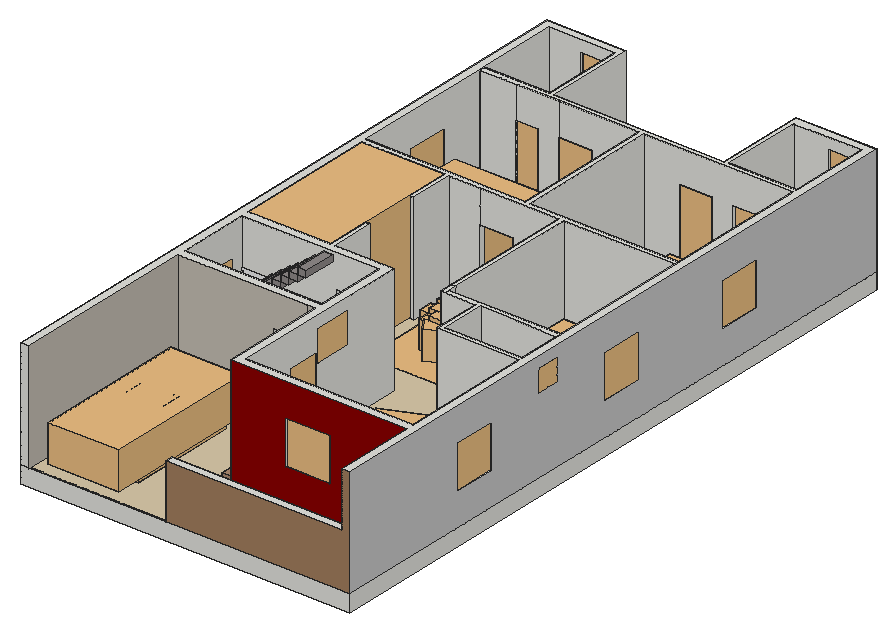
# SketchUp Ruby script. Lengths in inches.
U = 1.inch
M = Sketchup.active_model
def pt(a) = Geom::Point3d.new(a.map { |v| v * U })
def face(e, loops, mat)
  f = e.add_face(loops[0].map { |a| pt(a) })
  loops[1..].each { |l| e.add_face(l.map { |a| pt(a) }).erase! }
  f.material = f.back_material = mat if mat
  f
end
# faces: each face lists its corners as indices into pts; further lists are holes
def faces(e, pts, list, mat = nil) = list.each { |f| face(e, (f[0].is_a?(Array) ? f : [f]).map { |l| l.map { |i| pts[i] } }, mat) }
# xy, xz, yz: faces in a plane at the given z, y or x. An outline is a flat list of corners, or four numbers for a rectangle; further outlines are holes
def ring(l) = l.size == 4 ? [[l[0], l[1]], [l[2], l[1]], [l[2], l[3]], [l[0], l[3]]] : l.each_slice(2).to_a
def flat(e, list, mat, &to3) = list.each { |f| face(e, (f[0].is_a?(Array) ? f : [f]).map { |l| ring(l).map { |u, v| to3.(u, v) } }, mat) }
def xy(e, z, list, mat = nil) = flat(e, list, mat) { |x, y| [x, y, z] }
def xz(e, y, list, mat = nil) = flat(e, list, mat) { |x, z| [x, y, z] }
def yz(e, x, list, mat = nil) = flat(e, list, mat) { |y, z| [x, y, z] }
def lines(e, pts, list) = list.each { |a, b| e.add_line(pt(pts[a]), pt(pts[b])) }
# prism: a flat outline (further loops are holes) pulled along v
def prism(e, loops, v, mat = nil)
  f = face(e, loops, mat); d = Geom::Vector3d.new(v.map { |x| x * U })
  f.pushpull(f.normal.samedirection?(d) ? d.length : -d.length)
end
def box(e, o, s, mat = nil) = prism(e, [[o, [o[0] + s[0], o[1], o[2]], [o[0] + s[0], o[1] + s[1], o[2]], [o[0], o[1] + s[1], o[2]]]], [0, 0, s[2]], mat)
def at(x, y, z, deg = 0) = Geom::Transformation.translation(pt([x, y, z])) * Geom::Transformation.rotation(ORIGIN, Z_AXIS, deg.degrees)
def axes(o, x, y, z) = Geom::Transformation.new([*x, 0, *y, 0, *z, 0, *pt(o).to_a, 1])
def part(name) = M.definitions.add(name)
# library, detail: a bought-in or finely detailed component or shape, given as its bounding box
def library(name, o, s) = part(name).tap { |d| box(d.entities, o, s) }
def detail(e, o, s) = box(e.add_group.entities, o, s)
def put(e, d, t, mat = nil) = e.add_instance(d, t).tap { |i| i.material = mat if mat }
def group(e, t, mat = nil) = e.add_group.tap { |g| g.transformation = t; g.material = mat if mat }.entities
root = M.entities
M.materials.add("711 SAND (3).jpg").color = [199, 194, 187]
M.materials.add("Carpet_Saxony_Multi").color = [211, 205, 196]
M.materials.add("F40decal1").color = [13, 15, 14]
M.materials["F40decal1"].alpha = 0.5
M.materials.add("F40glass1").color = [81, 98, 101]
M.materials["F40glass1"].alpha = 0.5
M.materials.add("F40horse1").color = [80, 62, 2]
M.materials.add("F40oranB1").color = [93, 93, 93]
M.materials["F40oranB1"].alpha = 0.9
M.materials.add("F40pinin1").color = [154, 183, 194]
M.materials.add("F40pnl1").color = [44, 40, 40]
M.materials.add("F40pnl2").color = [46, 43, 49]
M.materials.add("F40pnl3").color = [69, 78, 80]
M.materials.add("F40shieF1").color = [153, 132, 60]
M.materials.add("Material~3").color = [234, 182, 87]
M.materials.add("[0021_DarkRed]").color = [139, 0, 0]
M.materials.add("[Aluminum]").color = [179, 179, 179]
M.materials.add("[Carrera Marble]").color = [207, 207, 207]
M.materials.add("[Cladding Siding Tan]").color = [162, 126, 95]
M.materials.add("[Cladding Stucco White]").color = [200, 200, 200]
M.materials.add("[Field Rectangle Tile]").color = [196, 189, 179]
M.materials.add("[Field Square Tile]").color = [217, 201, 169]
M.materials.add("[Metal Aluminum Anodized]").color = [202, 209, 219]
M.materials.add("[Square Glass Tile 01]").color = [211, 212, 216]
M.materials.add("[Stone Marble]").color = [143, 138, 136]
M.materials.add("[Tile Veriegated Stone]").color = [171, 137, 112]
M.materials.add("[Translucent_Glass_Blue]1").color = [100, 149, 237]
M.materials["[Translucent_Glass_Blue]1"].alpha = 0.5
M.materials.add("[sketch-stone]").color = [126, 99, 107]
M.materials.add("fear and loathing in las vegas").color = [238, 236, 236]
M.materials.add("first love last rites").color = [26, 26, 24]
c1 = library("BED",[11.85,23.38,0],[78.45,94.56,48.29])
c2 = library("rcv",[0,-1.57,0],[0.79,6.29,0.79])
c3 = library("Washing machine LG WD-80302NUP",[0,0,0],[18.43,23.62,33.46])
c4 = library("WALL MOUNTED TOILET",[-0.1,0,0],[25.85,37.27,34.47])
c5 = library("kpd",[0,0,0],[51.18,20.47,32.4375])
c6 = library("66666666666",[0,0,0],[67.875,28,18])
c7 = library("Armchair",[-16.34,-19.23,-0.05],[32.68,37.4,30.76])
c8 = library("Pillow-Alexandria[ID AX003]\#2",[-12.4,-4.05,0],[26.56,8.1,26.57])
c9 = library("VASO COM TULIPAS",[-1.0625,-0.96,-0.83],[20.78,20.79,25.09])
c10 = part("book - first love last rites")
g1 = group(c10.entities,at(-2.45,1.03,0,-90))
xy(g1,0,[[0,0,0,5.28,0.16,5.28,0.16,0.16,1.22,0.16,1.22,5.28,1.38,5.28,1.38,0]],"first love last rites")
xy(g1,0.08,[[0.16,0.16,1.22,5.2]])
xy(g1,7.8,[[0.16,0.16,1.22,5.2]])
xy(g1,7.875,[[0,0,1.38,0,1.38,5.28,1.22,5.28,1.22,0.16,0.16,0.16,0.16,5.28,0,5.28]],"first love last rites")
xz(g1,0,[[0,0,1.38,7.875]],"first love last rites")
xz(g1,0.16,[[0.16,0,1.22,0.08],[0.16,7.8,1.22,7.875]])
xz(g1,5.2,[[0.16,0.08,1.22,7.8]])
xz(g1,5.28,[[0,0,0.16,7.875],[1.22,0,1.38,7.875]],"first love last rites")
yz(g1,0,[[0,0,5.28,7.875]],"first love last rites")
yz(g1,0.16,[[0.16,0,5.28,0,5.28,7.875,0.16,7.875,0.16,7.8,5.2,7.8,5.2,0.08,0.16,0.08]])
yz(g1,1.22,[[0.16,0,0.16,0.08,5.2,0.08,5.2,7.8,0.16,7.8,0.16,7.875,5.28,7.875,5.28,0]])
yz(g1,1.38,[[0,0,5.28,7.875]],"first love last rites")
c11 = part("book - fear and loathing in las vegas")
g2 = group(c11.entities,at(-2.64,0.79,0,-90))
xy(g2,0,[[0,0,0,5.31,0.16,5.31,0.16,0.16,0.96,0.16,0.96,5.31,1.12,5.31,1.12,0]],"fear and loathing in las vegas")
xy(g2,0.08,[[0.16,0.16,0.96,5.24]])
xy(g2,7.8,[[0.16,0.16,0.96,5.24]])
xy(g2,7.875,[[0,0,1.12,0,1.12,5.31,0.96,5.31,0.96,0.16,0.16,0.16,0.16,5.31,0,5.31]],"fear and loathing in las vegas")
xz(g2,0,[[0,0,1.12,7.875]],"fear and loathing in las vegas")
xz(g2,0.16,[[0.16,0,0.96,0.08],[0.16,7.8,0.96,7.875]])
xz(g2,5.24,[[0.16,0.08,0.96,7.8]])
xz(g2,5.31,[[0,0,0.16,7.875]])
xz(g2,5.31,[[0.96,0,1.12,7.875]],"fear and loathing in las vegas")
yz(g2,0,[[0,0,5.31,7.875]],"fear and loathing in las vegas")
yz(g2,0.16,[[0.16,0,5.31,0,5.31,7.875,0.16,7.875,0.16,7.8,5.24,7.8,5.24,0.08,0.16,0.08]])
yz(g2,0.96,[[0.16,0,0.16,0.08,5.24,0.08,5.24,7.8,0.16,7.8,0.16,7.875,5.31,7.875,5.31,0]])
yz(g2,1.12,[[0,0,5.31,7.875]],"fear and loathing in las vegas")
c12 = library("SimLab",[-7.02,0.26,3.32],[7.24,1.79,7.15])
c13 = library("Round vase",[0,0,0],[4358.29,3919.47,3356.29])
c14 = library("Winged corkscrew",[-0.27,0,-0.18],[4.96,1.5,6.64])
c15 = library("Entrance door assembly",[0,0,0],[60,4,84])
c16 = part("d1")
xy(c16.entities,0,[[0,0,18,1.6],[18,0,36,1.6]],"[sketch-stone]")
xy(c16.entities,72,[[0,0,18,1.6],[18,0,36,1.6]],"[sketch-stone]")
yz(c16.entities,0,[[0,0,1.6,72]],"[sketch-stone]")
yz(c16.entities,36,[[0,0,1.6,72]],"[sketch-stone]")
c17 = library("porta 4",[0.2,-5.42,1.33],[46.55,4.72,83.21])
c18 = library("Door C1",[0,0,0],[35.43,8.39,80.71])
c19 = library("Entrance door assembly \#1",[0,0,0],[51.57,9.61,84.84])
c20 = library("ventilator",[0,0,0],[24,6.83,23.62])
c21 = library("F40belt",[-57.86,1.04,11.25],[71.2,11.3,17.75])
c22 = library("F40chrom",[-99.45,-166.43,-7.45],[154.35,313.83,56.55])
c23 = part("F40decal")
p = [[31.33,27.09,31.1875],[26.65,22.32,38.43],[31.99,20.9,30.8125],[26.29,22.41,38.92],[30.52,34.1,31.61],[26.04,22.49,39.35],
  [23.9375,49.76,38.48],[30.4,37.17,31.8]]
faces(c23.entities,p,[[0,1,2],[3,1,0],[0,4,3],[5,3,4],[6,5,4],[6,4,7]],"F40decal1")
c24 = library("F40dirty",[-53.11,44.58,-11.25],[61.59,105.73,37.89])
c25 = library("F40engB",[-48.82,62.57,25.53],[53.31,17.62,5.1])
c26 = library("F40engCH",[-71.65,25.73,-8.77],[98.75,110.76,40.52])
c27 = library("F40f40",[-100.37,-188.19,-24.03],[156.19,337.67,80.89])
c28 = library("F40glasB",[-61.58,-42.0625,46.26],[78.61,8.76,5.84])
c29 = part("F40horse")
p = [[-3.05,-53.51,15.1],[-4.57,-53.64,15.49],[-0.45,-53.96,16.52],[-1.53,-53.64,15.49],[-5.65,-53.96,16.52],[-4.57,-55.2,20.45],
  [-3.05,-55.32,20.84],[-1.53,-55.2,20.45],[-5.65,-54.875,19.42],[-0.45,-54.875,19.42],[-6.0625,-54.42,17.97],[-0.04,-54.42,17.97]]
faces(c29.entities,p,[[0,1,2],[3,0,2],[1,4,2],[5,6,2],[6,7,2],[8,5,2],[7,9,2],[10,8,2],
  [9,11,2],[4,10,2]],"F40horse1")
c30 = library("F40insid",[-76.73,-89.59,-18.91],[108.79,150.79,51.84])
c31 = library("F40lighG",[-85.29,-180.22,-1.74],[126.03,21.24,10.81])
c32 = part("F40lighL")
p = [[26.55,-166.03,4.41],[21.38,-166.36,4.41],[21.38,-166.41,-0.89],[26.55,-166.07,-0.89]]
faces(c32.entities,p,[[0,1,2],[0,2,3]],"F40glass1")
c33 = part("F40lighR")
p = [[-65.93,-166.36,4.41],[-71.1,-166.03,4.41],[-65.93,-166.41,-0.89],[-71.1,-166.07,-0.89]]
faces(c33.entities,p,[[0,1,2],[2,1,3]],"F40glass1")
c34 = library("F40net",[-85.48,-180.58,-18.99],[126.41,325.75,45.93])
c35 = library("F40netO",[-85.48,142.41,9.84],[126.41,2.73,17.1])
c36 = library("F40oran",[-95.36,-165.91,-0.52],[146.17,312.33,25.41])
c37 = part("F40oranB")
xz(c37.entities,146.42,[[-80.04,23.81,-76.4375,24.28,-75.32,23.81],[-80.04,23.81,-78.92,24.28,-76.4375,24.28],[30.77,23.81,31.88,24.28,35.49,23.81],[35.49,23.81,31.88,24.28,34.37,24.28],[-78.92,24.28,-77.68,24.45,-76.4375,24.28],
  [31.88,24.28,33.125,24.45,34.37,24.28]],"F40oranB1")
p = [[-80.77,-165.33,-0.5],[-71.9,-165.91,-0.48],[-80.77,-165.3,3.52],[-71.91,-165.875,3.54],[27.36,-165.8125,-0.48],[36.22,-165.43,-0.5],
  [36.21,-165.4,3.52],[27.35,-165.78,3.54],[-76.4375,146.34,15.26],[-77.68,146.34,15.09],[-80.99,146.41,23.08],[-78.92,146.34,15.26],
  [33.125,146.34,15.09],[31.88,146.34,15.26],[36.43,146.41,23.08],[34.37,146.34,15.26],[-75.32,146.35,15.73],[-80.04,146.35,15.73],
  [30.77,146.35,15.73],[35.49,146.35,15.73],[-74.375,146.35,16.46],[-80.99,146.35,16.46],[29.82,146.35,16.46],[36.43,146.35,16.46],
  [-81.72,146.36,17.41],[-73.64,146.36,17.41],[29.09,146.36,17.41],[37.17,146.36,17.41],[-82.19,146.37,18.53],[-73.17,146.37,18.53],
  [28.62,146.37,18.53],[37.64,146.37,18.53],[-82.36,146.38,19.77],[-73,146.38,19.77],[28.45,146.38,19.77],[37.8,146.38,19.77],
  [-82.19,146.39,21.01],[-73.17,146.39,21.01],[28.62,146.39,21.01],[37.64,146.39,21.01],[-81.72,146.4,22.13],[-73.64,146.4,22.13],
  [29.09,146.4,22.13],[37.17,146.4,22.13],[-74.375,146.41,23.08],[29.82,146.41,23.08],[-80.04,146.42,23.81],[-75.32,146.42,23.81],
  [30.77,146.42,23.81],[35.49,146.42,23.81]]
faces(c37.entities,p,[[0,1,2],[2,1,3],[4,5,6],[4,6,7],[8,9,10],[9,11,10],[12,13,14],[15,12,14],
  [16,8,10],[11,17,10],[13,18,14],[19,15,14],[20,16,10],[17,21,10],[18,22,14],[23,19,14],
  [21,24,10],[25,20,10],[22,26,14],[27,23,14],[24,28,10],[29,25,10],[26,30,14],[31,27,14],
  [28,32,10],[33,29,10],[30,34,14],[35,31,14],[32,36,10],[37,33,10],[34,38,14],[39,35,14],
  [36,40,10],[41,37,10],[38,42,14],[43,39,14],[44,41,10],[42,45,14],[46,44,10],[47,44,46],
  [45,48,49],[45,49,14]],"F40oranB1")
c38 = part("F40pinin")
p = [[-96.35,47.75,5.21],[-97.17,55.16,6.91],[-97.32,55.14,5.23],[-96.19,47.76,6.88],[52.625,55.16,6.91],[51.64,47.76,6.88],
  [51.8,47.75,5.21],[52.77,55.14,5.23]]
faces(c38.entities,p,[[0,1,2],[3,1,0],[4,5,6],[4,6,7]],"F40pinin1")
c39 = library("F40pirel",[-98.14,-129.17,-31.36],[151.73,236.53,47.57])
c40 = library("F40plstc",[-98.3125,-185.14,-24.34],[152.07,333.62,79.49])
c41 = part("F40pnl1")
detail(c41.entities,[-11.32,-69.72,18.98],[21.44,0.94,10.49])
c42 = part("F40pnl2")
p = [[-35.57,-67.49,23.09],[-14.75,-67.54,17.64],[-35.57,-67.54,17.64],[-14.75,-67.49,23.09]]
faces(c42.entities,p,[[0,1,2],[3,1,0]],"F40pnl2")
c43 = part("F40pnl3")
p = [[-67.72,-67.07,24.13],[-38.78,-67.17,12.25],[-67.72,-67.17,12.25],[-38.78,-67.07,24.13]]
faces(c43.entities,p,[[0,1,2],[3,1,0]],"F40pnl3")
c44 = library("F40seat",[-67.14,-36.68,-16.68],[89.79,54.9,59.25])
c45 = library("F40seatB",[-62.47,-25.49,-14.85],[80.44,48.57,70.03])
c46 = part("F40shieF")
p = [[-24.09,-182.11,-1.4375],[-22.28,-182.11,-1.43],[-22.28,-178.32,0.9],[-24.09,-179.08,0.43],[-20.46,-179.08,0.43],[-20.46,-182.11,-1.4375],
  [-24.09,-178.01,1.07],[-20.46,-178.01,1.07],[-24.09,-174.92,2.89],[-22.28,-174.92,2.9],[-20.46,-174.92,2.89]]
faces(c46.entities,p,[[0,1,2],[2,3,0],[4,2,1],[1,5,4],[3,2,6],[7,2,4],[8,6,2],[2,9,8],
  [2,7,10],[10,9,2]],"F40shieF1")
c47 = library("F40shieS",[-95.33,-80.8,15.58],[146.11,6.87,9.3])
c48 = library("F40stop",[-70.83,143.73,15.12],[97.11,2.7,10.21])
c49 = library("F40stopB",[-70.41,146.34,15.54],[96.27,0.09,9.35])
c50 = library("F40tire",[-97.86,-130.55,-32.75],[151.17,239.6,50.41])
c51 = library("F40wdowB",[-66.31,48.18,32.68],[88.07,75.29,19.68])
c52 = library("F40wdowF",[-72.23,-88.02,28.55],[99.91,45.99,20.53])
c53 = part("F40wdowL")
detail(c53.entities,[18.73,20.9,30.8125],[12.92,30.54,18.0625])
c54 = part("F40wdowM")
detail(c54.entities,[-61.41,38.83,25.72],[78.27,21.54,22.47])
c55 = part("F40wdowR")
detail(c55.entities,[-76.2,20.9,30.8125],[12.92,30.54,18.0625])
c56 = library("F40whlC",[-97.96,-125.09,-27.3],[151.37,228.23,39.24])
c57 = part("Ferrari F40")
put(c57.entities,c21,at(0,0,0))
put(c57.entities,c22,at(0,0,0))
put(c57.entities,c23,at(0,0,0))
put(c57.entities,c24,at(0,0,0))
put(c57.entities,c25,at(0,0,0))
put(c57.entities,c26,at(0,0,0))
put(c57.entities,c27,at(0,0,0))
put(c57.entities,c28,at(0,0,0))
put(c57.entities,c29,at(0,0,0))
put(c57.entities,c30,at(0,0,0))
put(c57.entities,c31,at(0,0,0))
put(c57.entities,c32,at(0,0,0))
put(c57.entities,c33,at(0,0,0))
put(c57.entities,c34,at(0,0,0))
put(c57.entities,c35,at(0,0,0))
put(c57.entities,c36,at(0,0,0))
put(c57.entities,c37,at(0,0,0))
put(c57.entities,c38,at(0,0,0))
put(c57.entities,c39,at(0,0,0))
put(c57.entities,c40,at(0,0,0))
put(c57.entities,c41,at(0,0,0))
put(c57.entities,c42,at(0,0,0))
put(c57.entities,c43,at(0,0,0))
put(c57.entities,c44,at(0,0,0))
put(c57.entities,c45,at(0,0,0))
put(c57.entities,c46,at(0,0,0))
put(c57.entities,c47,at(0,0,0))
put(c57.entities,c48,at(0,0,0))
put(c57.entities,c49,at(0,0,0))
put(c57.entities,c50,at(0,0,0))
put(c57.entities,c51,at(0,0,0))
put(c57.entities,c52,at(0,0,0))
put(c57.entities,c53,at(0,0,0))
put(c57.entities,c54,at(0,0,0))
put(c57.entities,c55,at(0,0,0))
put(c57.entities,c56,at(0,0,0))
c58 = part("skeF529")
put(c58.entities,c57,at(-22.68,64.14,-12.05))
c59 = part("Bez")
p = [[6.61,40.01,0.09],[4.18,40.02,0.08],[4.2,42.375,1.11],[23.74,30.58,-3.93],[25.22,34.3,-2.29],[25.6,38.25,-0.56],
  [24.85,42.16,1.15],[23.02,45.76,2.71],[20.24,48.81,4.03],[16.69,51.1,5],[12.625,52.46,5.58],[8.3125,52.82,5.71],
  [4.05,52.14,5.39],[0.12,50.48,4.63],[-3.2,47.94,3.5],[-5.68,44.69,2.07],[-7.17,40.97,0.43],[-7.54,37.02,-1.3],
  [-6.79,33.11,-3.01],[-4.97,29.51,-4.57],[-2.18,26.46,-5.89],[1.36,24.18,-6.87],[5.43,22.81,-7.44],[9.74,22.45,-7.57],
  [14.01,23.13,-7.25],[17.93,24.8,-6.49],[21.25,27.34,-5.36],[4.15,34.02,-2.54],[10.03,36.65,-1.36]]
faces(c59.entities,p,[[0,1,2]])
lines(c59.entities,p,[[3,4],[4,5],[5,6],[6,7],[7,8],[8,9],[9,10],[10,11],[11,12],[12,13],[13,14],[14,15],
  [15,16],[16,17],[17,18],[18,19],[19,20],[20,21],[21,22],[22,23],[23,24],[24,25],[25,26],[26,3],
  [1,27],[0,28]])
put(c59.entities,c58,at(60.36,131,0))
c60 = part("Group4678\#1")
box(c60.entities,[279.51,732.57,0],[2.36,2.36,41.54])
c61 = part("Group4679\#1")
box(c61.entities,[93.51,732.57,0],[2.36,2.36,41.54])
c62 = part("Group4680\#1")
box(c62.entities,[233.6,732.57,0],[1.18,2.36,41.54])
box(c62.entities,[187.1,732.57,0],[1.18,2.36,41.54])
box(c62.entities,[140.6,732.57,0],[1.18,2.36,41.54])
c63 = part("Group4681\#1")
box(c63.entities,[93.51,732.37,41.54],[188.36,2.76,1.77])
c64 = part("Group4682\#1")
box(c64.entities,[94.6875,732.77,36.42],[186,1.96,0.99])
c65 = part("Group4683\#1")
box(c65.entities,[94.6875,732.77,4.92],[186,1.96,0.99])
c66 = part("Group4684\#1")
xz(c66.entities,733.75,[[94.6875,5.91,280.6875,36.42]],"[Translucent_Glass_Blue]1")
c67 = part("Group\#6")
box(c67.entities,[0,0,0],[9.43,36,7])
c68 = part("Group\#7")
box(c68.entities,[0,0,0],[9.43,36,7])
c69 = library("Group\#59",[0,0,0],[107.09,109.45,86.61])
c70 = library("组\#36",[0,0,0],[63.98,38.52,35.22])
c71 = library("组\#212",[0,0,0],[26.5625,8.1,26.57])
c72 = library("Groupe\#2",[0,0,0],[128.09,128.09,227.02])
c73 = library("组\#93",[0,0,0],[23.62,23.62,23.62])
c74 = library("组\#211",[0,0,0],[26.5625,8.1,26.57])
c75 = library("Group\#84",[0,0,0],[74.75,0.57,42.04])
c76 = library("组\#78",[0,0,0],[23.62,23.62,23.62])
c77 = library("Grouper\#1",[0,0,0],[11.8125,11.8125,21.26])
c78 = library("组\#246",[0,1.1,0],[38.58,108.89,33.46])
c79 = part("组\#198")
box(c79.entities,[32.99,7.44,0],[108.66,131.06,0.2])
c80 = library("Agrupar\#70",[0,0,0],[34.17,1.77,47.95])
c81 = library("Agrupar\#69",[0,0,0],[34.17,1.77,47.95])
c82 = library("Grupo\#24",[0,0,0],[8.03,7.94,3.08])
c83 = library("Grupo\#25",[0,0,0],[12.75,12.75,9.37])
c84 = library("Agrupar\#65",[-2.07,-2.97,0],[25.13,25.12,18.375])
c85 = library("建立群組\#1",[-0.2,-1.22,-0.05],[8.68,4.74,2.11])
c86 = library("Grupo\#11",[0,0,-0.16],[14.35,15.43,6.36])
c87 = library("Grupo\#10",[0,0,0],[78.88,39.54,29.55])
c88 = library("Group\#304",[-0.05,-0.14,-0.21],[19.14,22.42,31.43])
c89 = library("Group\#207",[-0.05,-0.14,-0.21],[19.14,22.42,31.43])
c90 = library("Group\#208",[0,0,0],[78.74,114.17,0.59])
c91 = library("Grupo\#160",[0,0,0],[13.78,78.74,32.28])
c92 = library("Grupo\#20",[-0.22,-0.18,0],[9.04,9.89,23.41])
c93 = library("Group\#472",[0,0,0],[117.98,117.98,518.53])
c94 = library("Group\#206",[0,0,0],[6.59,5.55,7.5])
c95 = part("Agrupar\#10")
prism(c95.entities,[[[59.06,0,0],[0,0,0],[0,94.49,0],[59.06,94.49,0],[68.9,94.49,0],[68.9,9.84,0],[68.9,0,0]]],[0,0,1.18])
c96 = library("Group\#371",[0,0,-1.18],[130.86,88.125,32.92])
c97 = library("Group\#428",[0,-25,0],[5.5,114,60])
xy(root,0,[[101.57,255,111,291]])
xy(root,7.4,[[181.22,98.03,351,242]])
xy(root,17.64,[[275.02,247,351,247,351,279.14,341.94,279.14,341.94,295,275.02,295],[7,635.02,81,635.02,81,711,31.45,711,31.45,701.94,7,701.94],[277,635.02,351,635.02,351,711,301.45,711,301.45,701.94,277,701.94]],"[Square Glass Tile 01]")
xy(root,66.46,[[275.02,247,275.02,252.36,288.8,252.36,288.8,247.43,337.22,247.43,337.22,252.36,351,252.36,351,247],[72.74,635.02,72.74,648.8,80.34,648.8,80.34,697.22,72.74,697.22,72.74,711,81,711,81,635.02],[342.74,635.02,342.74,648.8,350.34,648.8,350.34,697.22,342.74,697.22,342.74,711,351,711,351,635.02]])
xy(root,106.22,[[288.8,247.43,337.22,252.36],[72.74,648.8,80.34,697.22],[342.74,648.8,350.34,697.22]])
xy(root,107.01,[[275.8,247,350.21,250.86],[275.02,251.29,351,252.36],[72.74,635.02,74.39,711],[342.74,635.02,344.39,711],[75.05,635.8,81,710.21],
  [345.05,635.8,351,710.21]])
xy(root,109.76,[[275.02,247,275.8,250.86],[350.21,247,351,250.86],[275.02,250.86,351,251.29],[74.39,635.02,75.05,711],[75.05,635.02,81,635.8],
  [344.39,635.02,345.05,711],[345.05,635.02,351,635.8],[75.05,710.21,81,711],[345.05,710.21,351,711]])
xz(root,247,[[275.02,66.46,351,66.46,351,109.76,350.21,109.76,350.21,107.01,275.8,107.01,275.8,109.76,275.02,109.76]])
xz(root,247,[[275.02,17.64,351,66.46]],"[Square Glass Tile 01]")
xz(root,247.43,[[288.8,66.46,337.22,106.22]],"[Metal Aluminum Anodized]")
xz(root,250.86,[[275.8,107.01,350.21,109.76]])
xz(root,251.29,[[275.02,107.01,351,109.76]])
xz(root,252.36,[[275.02,66.46,275.8,106.22],[275.8,66.46,288.01,106.22],[288.01,66.46,288.8,106.22],[337.22,66.46,338.01,106.22],[338.01,66.46,350.21,106.22],
  [350.21,66.46,351,106.22],[275.02,106.22,351,107.01]])
xz(root,635.02,[[72.74,66.46,81,106.22],[342.74,66.46,351,106.22],[72.74,106.22,81,107.01],[342.74,106.22,351,107.01],[74.39,107.01,81,109.76],
  [344.39,107.01,351,109.76]])
xz(root,635.8,[[75.05,107.01,81,109.76],[345.05,107.01,351,109.76]])
xz(root,648.8,[[72.74,66.46,80.34,106.22],[342.74,66.46,350.34,106.22]])
xz(root,697.22,[[72.74,66.46,80.34,106.22],[342.74,66.46,350.34,106.22]])
xz(root,710.21,[[75.05,107.01,81,109.76],[345.05,107.01,351,109.76]])
xz(root,711,[[72.74,66.46,72.74,107.01,74.39,107.01,74.39,109.76,81,109.76,81,66.46],[342.74,66.46,342.74,107.01,344.39,107.01,344.39,109.76,351,109.76,351,66.46]])
yz(root,72.74,[[635.02,66.46,635.8,106.22],[635.8,66.46,648.01,106.22],[648.01,66.46,648.8,106.22],[697.22,66.46,698.01,106.22],[698.01,66.46,710.21,106.22],
  [710.21,66.46,711,106.22],[635.02,106.22,711,107.01]])
yz(root,74.39,[[635.02,107.01,711,109.76]])
yz(root,75.05,[[635.8,107.01,710.21,109.76]])
yz(root,80.34,[[648.8,66.46,697.22,106.22]],"[Metal Aluminum Anodized]")
yz(root,81,[[635.02,66.46,711,66.46,711,109.76,710.21,109.76,710.21,107.01,635.8,107.01,635.8,109.76,635.02,109.76]])
yz(root,81,[[635.02,17.64,711,66.46],[635.8,107.01,635.8,109.76,635.02,109.76,635.02,120,711,120,711,109.76,710.21,109.76,710.21,107.01]],"[Square Glass Tile 01]")
yz(root,275.02,[[247,66.46,252.36,106.22],[247,106.22,252.36,107.01],[247,107.01,251.29,109.76]])
yz(root,275.8,[[247,107.01,250.86,109.76]])
yz(root,288.8,[[247.43,66.46,252.36,106.22]])
yz(root,337.22,[[247.43,66.46,252.36,106.22]])
yz(root,342.74,[[635.02,66.46,635.8,106.22],[635.8,66.46,648.01,106.22],[648.01,66.46,648.8,106.22],[697.22,66.46,698.01,106.22],[698.01,66.46,710.21,106.22],
  [710.21,66.46,711,106.22],[635.02,106.22,711,107.01]])
yz(root,344.39,[[635.02,107.01,711,109.76]])
yz(root,345.05,[[635.8,107.01,710.21,109.76]])
yz(root,350.21,[[247,107.01,250.86,109.76]])
yz(root,350.34,[[648.8,66.46,697.22,106.22]],"[Metal Aluminum Anodized]")
yz(root,351,[[247,66.46,252.36,66.46,252.36,107.01,251.29,107.01,251.29,109.76,247,109.76],[635.02,66.46,711,66.46,711,109.76,710.21,109.76,710.21,107.01,635.8,107.01,635.8,109.76,635.02,109.76]])
yz(root,351,[[635.02,17.64,711,66.46],[635.8,107.01,635.8,109.76,635.02,109.76,635.02,120,711,120,711,109.76,710.21,109.76,710.21,107.01]],"[Square Glass Tile 01]")
p = [[9,9,120],[9,0,120],[9,0,0],[9,213,49],[45,252,49],[9,291,49],
  [9,252,49],[267,247,120],[273,247,120],[273,315,121],[273.0625,315,121],[273,285,121],
  [273.0625,285,121],[275.02,247,109.76],[275.02,247,120],[351,247,109.76],[351,247,120],[351,279.14,120],
  [7,701.94,17.64],[7,701.94,120],[-59.64,1991.54,1.35],[-59.5,1991.66,1.36],[-73.67,1987.46,56.89],[-73.8,1987.57,57.05],
  [-67.95,1988.53,57],[-67.8,1988.59,57.16],[-69.79,1983.17,56.96],[-69.82,1983.01,57.12],[-78.78,1992.37,1],[-78.96,1992.4375,1],
  [-69.94,1975.38,1.16],[-69.91,1975.2,1.16]]
lines(root,p,[[0,1],[1,2],[3,4],[4,5],[4,6],[7,8],[9,10],[11,12],[13,14],[15,16],[14,16],[16,17],
  [18,19],[20,21],[22,23],[24,25],[26,27],[28,29],[30,31]])
put(root,c1,at(126.9375,491.59,0,90))
put(root,c1,at(233.0625,578.8,0,-90))
put(root,c1,at(233.0625,433.49,0,-90))
put(root,c2,axes([283.37,252.36,67.85],[0,0.54429,0],[-1,0,0],[0,0,1]))
put(root,c3,axes([298.64,248.01,17.64],[0,0.54429,0],[-1,0,0],[0,0,1]))
put(root,c4,axes([351,270.2,27.43],[0,0.27759,0],[-0.51,0,0],[0,0,0.51]))
put(root,c5,axes([351,258.14,31.42],[-1,0,0],[0,-0.54429,0],[0,0,1]))
put(root,c2,axes([345.57,252.36,67.85],[0,0.54429,0],[-1,0,0],[0,0,1]))
put(root,c2,axes([72.74,643.37,67.85],[-0.83911,0,0],[0,-1,0],[0,0,1]))
put(root,c3,axes([79.45,658.64,17.64],[-0.83911,0,0],[0,-1,0],[0,0,1]))
put(root,c6,axes([7,701.94,17.64],[0,-0.98608,0],[0.87309,0,0],[0,0,1]))
put(root,c4,axes([54.99,711,17.64],[-0.42794,0,0],[0,-0.51,0],[0,0,0.51]))
put(root,c5,axes([63.82,711,31.42],[0,-1,0],[0.83911,0,0],[0,0,1]))
put(root,c2,axes([72.74,705.57,67.85],[-0.83911,0,0],[0,-1,0],[0,0,1]))
put(root,c2,axes([342.74,643.37,67.85],[-0.83911,0,0],[0,-1,0],[0,0,1]))
put(root,c3,axes([349.45,658.64,17.64],[-0.83911,0,0],[0,-1,0],[0,0,1]))
put(root,c6,axes([277,701.94,17.64],[0,-0.98608,0],[0.87309,0,0],[0,0,1]))
put(root,c4,axes([320.88,711,17.67],[-0.42794,0,0],[0,-0.51,0],[0,0,0.51]))
put(root,c5,axes([333.82,711,31.42],[0,-1,0],[0.83911,0,0],[0,0,1]))
put(root,c2,axes([342.74,705.57,67.85],[-0.83911,0,0],[0,-1,0],[0,0,1]))
put(root,c7,axes([271.68,120.76,7.65],[-0.88105,0,0],[0,-0.6649,0],[0,0,1]))
put(root,c8,axes([307.32,183.41,23.46],[0.55554,-0.24644,0.0117],[0.53485,0.67999,-0.31778],[0.06978,0.10325,0.65107]))
put(root,c8,axes([309.3,140.36,23.46],[-0.56057,-0.23986,0.0117],[0.51291,-0.68955,-0.31778],[0.0836,-0.09723,0.65107]))
put(root,c9,axes([252.45,150.5625,24.38],[0,0.51795,0],[-0.68634,0,0],[0,0,0.779]))
put(root,c7,axes([237.89,120.76,7.65],[-0.88105,0,0],[0,-0.6649,0],[0,0,1]))
put(root,c10,axes([250.6875,169.37,25.64],[0,0.6649,0],[0,0,-1],[0.88105,0,0]))
put(root,c11,axes([251.91,166.8,26.87],[-0.623,0.47015,0],[0,0,-1],[0.623,0.47015,0]))
put(root,c12,axes([215.36,406.89,25.35],[1.11,0,0],[0,0,1.11],[0,-1.8315,0]))
put(root,c13,axes([209.92,368.48,30.68],[0,-0.0017,0],[0.0017,0,0],[0,0,0.0034]))
put(root,c14,axes([157.65,403.7,29.95],[-0.72726,0.45567,0],[0,0,1],[0.51302,0.64595,0]))
put(root,c15,axes([114,206.4,0],[0.6,0,0],[0,1,0],[0,0,1]))
put(root,c16,axes([113,294.4375,0],[1.02778,0,0],[0,2.3625,0],[0,0,1.16667]))
put(root,c16,axes([138,456,0],[1,0,0],[0,2.3625,0],[0,0,1.16667]))
put(root,c16,axes([188,456,0],[1,0,0],[0,3.125,0],[0,0,1.16667]))
put(root,c16,axes([229,309,0],[0,1,0],[-3.125,0,0],[0,0,1.16667]))
put(root,c17,axes([226.84,622.42,-1.33],[0.77339,0,0],[0,1,0],[0,0,1]))
put(root,c17,axes([94.84,622.42,-1.33],[0.77339,0,0],[0,1,0],[0,0,1]))
put(root,c18,axes([48,618.72,0],[0.67733,0,0],[0,0.25502,0],[0,0,1.04078]))
put(root,c18,axes([286,618.72,0],[0.67733,0,0],[0,0.25502,0],[0,0,1.0403]))
put(root,c18,axes([263.8125,286,0],[0,-0.67733,0],[0.25502,0,0],[0,0,1.0404]))
put(root,c19,axes([166.54,107,0],[0,0.69802,0],[-0.78378,0,0],[0,0,1]))
put(root,c20,at(360,259,84,90))
put(root,c20,at(339,720,84,180))
put(root,c20,at(68,720,84,180))
put(root,c59,axes([52.42,7.3,22.32],[0.4982,0,0],[0,0.4982,0],[0,0,0.4982]))
g3 = group(root,at(45,213,0))
p = [[28.29,36,0],[28.29,0,0],[66,36,0],[66,42,0],[0,36,0],[0,42,0],
  [37.71,42,0],[37.71,57.94,0],[28.29,42,0],[28.29,57.94,0],[47.14,36,0],[56.57,36,0],
  [18.86,42,0],[18.86,57.94,0],[0,78,0],[9.43,42,0],[9.43,57.94,0],[37.71,36,0],
  [37.71,0,0],[0,0,0],[9.43,36,0],[9.43,0,0],[56.57,42,0],[56.57,57.94,0],
  [47.14,42,0],[47.14,57.94,0],[56.57,0,0],[47.14,0,0],[18.86,36,0],[47.14,78,0],
  [9.43,78,0],[56.57,78,0],[18.86,78,0],[37.71,78,0],[28.29,78,0],[66,78,0],
  [18.86,0,0]]
lines(g3,p,[[0,1],[2,3],[4,5],[6,7],[8,9],[10,11],[12,13],[11,2],[5,14],[15,16],[17,18],[19,4],
  [20,21],[5,15],[22,23],[24,25],[11,26],[10,27],[28,0],[25,29],[16,30],[17,10],[0,17],[23,31],
  [13,32],[20,28],[7,33],[9,34],[6,24],[24,22],[22,3],[3,35],[15,12],[12,8],[8,6],[28,36],
  [4,20]])
g4 = group(root,at(0,0,-18))
xy(g4,0,[[0,0,360,720]])
xy(g4,18,[[[0,0,360,720],[2,2,358,718]],[2,2,358,718]],"[Field Square Tile]")
xz(g4,0,[[0,0,360,18]])
xz(g4,720,[[0,0,360,18]])
yz(g4,0,[[0,0,720,18]])
yz(g4,360,[[0,0,720,18]])
put(g4,c60,at(-8.6875,-15.75,18))
put(g4,c61,at(-8.6875,-15.75,18))
put(g4,c62,at(-8.6875,-15.75,18),"[Aluminum]")
put(g4,c63,at(-8.6875,-15.75,18),"[Aluminum]")
put(g4,c64,at(-8.6875,-15.75,18),"[Aluminum]")
put(g4,c65,at(-8.6875,-15.75,18),"[Aluminum]")
put(g4,c66,at(-8.6875,-15.75,18))
g5 = group(root,at(111,89,0),"[Tile Veriegated Stone]")
prism(g5,[[[38,105,0],[0,105,0],[0,115,0],[48,115,0],[48,0,0],[38,0,0]]],[0,0,6])
put(root,c67,at(92.14,213,0),"[Stone Marble]")
put(root,c67,at(82.71,213,7),"[Stone Marble]")
put(root,c67,at(73.29,213,14),"[Stone Marble]")
put(root,c67,at(63.86,213,21),"[Stone Marble]")
put(root,c67,at(54.43,213,28),"[Stone Marble]")
put(root,c67,at(45,213,35),"[Stone Marble]")
g6 = group(root,at(35.57,213,42),"[Carrera Marble]")
xy(g6,0,[[-26.57,0,9.43,78]])
xy(g6,7,[[-26.57,0,9.43,0,9.43,39]])
xy(g6,14,[[-26.57,0,9.43,39,-26.57,39]])
xy(g6,21,[[-26.57,39,9.43,39,-26.57,78]])
xy(g6,28,[[9.43,39,9.43,78,-26.57,78]])
xz(g6,0,[[-26.57,0,9.43,7]])
xz(g6,39,[[-26.57,14,9.43,21]])
xz(g6,78,[[-26.57,0,9.43,28]])
yz(g6,-26.57,[[0,0,0,14,39,14,39,21,78,21,78,0]])
yz(g6,9.43,[[0,0,78,0,78,28,39,28,39,7,0,7]])
p = [[-26.57,0,7],[9.43,39,7],[9.43,39,14],[-26.57,0,14],[-26.57,78,21],[9.43,39,21],
  [9.43,39,28],[-26.57,78,28]]
faces(g6,p,[[0,1,2,3],[4,5,6,7]])
put(root,c68,at(45,252,70),"[Stone Marble]")
put(root,c68,at(54.43,252,77),"[Stone Marble]")
put(root,c68,at(63.86,252,84),"[Stone Marble]")
put(root,c68,at(73.29,252,91),"[Stone Marble]")
put(root,c68,at(82.71,252,98),"[Stone Marble]")
put(root,c68,at(92.14,252,105),"[Stone Marble]")
put(root,c68,at(101.57,252,112),"[Stone Marble]")
g7 = group(root,at(0,0,0))
xy(g7,0,[[0,0,0,720,86,720,86,622,95,622,95,617,72,617,72,622,81,622,81,711,9,711,9,461,138,461,138,456,104,456,104,408,99,408,99,456,9,456,9,300,99,300,99,348,104,348,104,300,113,300,113,291,9,291,9,213,114,213,114,204,9,204,9,0],[159,0,159,9,351,9,351,89,159,89,159,107,168,107,168,98,351,98,351,242,262,242,262,262,267,262,267,247,351,247,351,617,310,617,310,622,351,622,351,711,277,711,277,622,286,622,286,617,263,617,263,622,272,622,272,720,360,720,360,0],[159,143,159,204,150,204,150,213,159,213,159,291,150,291,150,300,168,300,168,143],[262,286,262,295,229,295,229,300,351,300,351,295,267,295,267,286],[224,345,224,461,351,461,351,456,229,456,229,345],
  [174,456,174,461,183,461,183,617,131,617,131,622,227,622,227,617,188,617,188,456],[9,617,48,622]])
xy(g7,36,[[219,89,267,98],[351,146,360,194],[159,159,168,195],[0,231,9,279],[351,348,360,396],
  [0,360,9,408],[351,508.68,360,556.68],[0,521,9,569]])
xy(g7,60,[[159,0,351,9]])
xy(g7,84,[[219,89,267,98],[159,107,168,143],[351,146,360,194],[159,159,168,195],[114,204,150,213],
  [0,231,9,279],[351,259,360,283],[262,262,267,286],[113,291,150,300],[224,309,229,345],
  [351,348,360,396],[0,360,9,408],[138,456,174,461],[188,456,224,461],[351,508.68,360,556.68],
  [0,521,9,569],[48,617,72,622],[95,617,131,622],[227,617,263,622],[286,617,310,622],
  [44,711,68,720],[315,711,339,720]])
xy(g7,108,[[351,259,360,283],[44,711,68,720],[315,711,339,720]])
xy(g7,120,[[[0,0,9,0,9,204,159,204,159,89,351,89,351,0,360,0,360,720,272,720,272,622,86,622,86,720,0,720],[168,98,168,300,104,300,104,348,99,348,99,300,9,300,9,456,99,456,99,408,104,408,104,456,138,456,138,461,9,461,9,711,81,711,81,622,9,622,9,617,183,617,183,461,138,461,138,456,224,456,224,309,229,309,229,456,351,456,351,461,188,461,188,617,351,617,351,247,267,247,267,295,351,295,351,300,229,300,229,295,262,295,262,242,351,242,351,98],[9,213,159,291],[277,622,351,711]],[224,295,229,309]])
xz(g7,0,[[0,0,9,120]])
xz(g7,0,[[159,0,360,0,360,120,351,120,351,60,159,60]],"[Cladding Siding Tan]")
xz(g7,9,[[159,0,351,60]])
xz(g7,89,[[[159,0,351,120],[219,36,267,84]]],"[0021_DarkRed]")
xz(g7,98,[[[168,0,351,120],[219,36,267,84]]])
xz(g7,107,[[159,0,168,84]])
xz(g7,143,[[159,0,168,84]])
xz(g7,146,[[351,36,360,84]])
xz(g7,159,[[159,36,168,84]])
xz(g7,194,[[351,36,360,84]])
xz(g7,195,[[159,36,168,84]])
xz(g7,204,[[9,0,114,0,114,84,150,84,150,120,9,120],[150,0,159,120]],"[Field Rectangle Tile]")
xz(g7,213,[[9,0,9,120,159,120,159,0,150,0,150,84,114,84,114,0]])
xz(g7,231,[[0,36,9,84]])
xz(g7,242,[[262,0,351,120]])
xz(g7,247,[[267,0,351,120]])
xz(g7,259,[[351,84,360,108]])
xz(g7,262,[[262,0,267,84]])
xz(g7,279,[[0,36,9,84]])
xz(g7,283,[[351,84,360,108]])
xz(g7,286,[[262,0,267,84]])
xz(g7,291,[[9,0,113,0,113,84,150,84,150,0,159,0,159,120,9,120]])
xz(g7,295,[[224,0,262,120],[267,0,351,120]])
xz(g7,300,[[9,0,99,120],[104,0,104,120,168,120,168,0,150,0,150,84,113,84,113,0],[229,0,351,120]])
xz(g7,309,[[224,0,229,84]])
xz(g7,345,[[224,0,229,84]])
xz(g7,348,[[99,0,104,120],[351,36,360,84]])
xz(g7,360,[[0,36,9,84]])
xz(g7,396,[[351,36,360,84]])
xz(g7,408,[[99,0,104,120],[0,36,9,84]])
xz(g7,456,[[9,0,99,120],[104,0,138,120],[174,0,188,0,188,84,224,84,224,120,138,120,138,84,174,84],[229,0,351,120]])
xz(g7,461,[[9,0,138,120],[174,0,174,84,138,84,138,120,183,120,183,0],[224,0,224,84,188,84,188,120,351,120,351,0]])
xz(g7,508.68,[[351,36,360,84]])
xz(g7,521,[[0,36,9,84]])
xz(g7,556.68,[[351,36,360,84]])
xz(g7,569,[[0,36,9,84]])
xz(g7,617,[[9,0,48,120],[72,0,95,0,95,120,48,120,48,84,72,84],[131,0,183,0,183,120,95,120,95,84,131,84],[188,0,227,0,227,84,263,84,263,0,286,0,286,84,310,84,310,0,351,0,351,120,188,120]])
xz(g7,622,[[9,0,9,120,81,120,81,0,72,0,72,84,48,84,48,0],[86,0,86,120,272,120,272,0,263,0,263,84,227,84,227,0,131,0,131,84,95,84,95,0],[277,0,277,120,351,120,351,0,310,0,310,84,286,84,286,0]])
xz(g7,711,[[[9,0,81,120],[44,84,68,108]],[[277,0,351,120],[315,84,339,108]]])
xz(g7,720,[[[0,0,86,120],[44,84,68,108]],[[272,0,360,120],[315,84,339,108]]],"[Cladding Stucco White]")
yz(g7,0,[[[0,0,720,120],[231,36,279,84],[360,36,408,84],[521,36,569,84]]],"[Cladding Stucco White]")
yz(g7,9,[[[213,0,291,120],[231,36,279,84]],[[300,0,456,120],[360,36,408,84]],[[461,0,617,120],[521,36,569,84]],[617,0,622,120],[622,0,711,120]])
yz(g7,9,[[0,0,204,120]],"[Field Rectangle Tile]")
yz(g7,44,[[711,84,720,108]])
yz(g7,48,[[617,0,622,84]])
yz(g7,68,[[711,84,720,108]])
yz(g7,72,[[617,0,622,84]])
yz(g7,81,[[622,0,711,120]])
yz(g7,86,[[622,0,720,120]])
yz(g7,95,[[617,0,622,84]])
yz(g7,99,[[300,0,348,120],[408,0,456,120]])
yz(g7,104,[[300,0,348,120],[408,0,456,120]])
yz(g7,113,[[291,0,300,84]])
yz(g7,114,[[204,0,213,84]])
yz(g7,131,[[617,0,622,84]])
yz(g7,138,[[456,0,461,84]])
yz(g7,150,[[204,0,213,84],[291,0,300,84]])
yz(g7,159,[[0,0,9,60],[[89,0,89,120,204,120,204,0,143,0,143,84,107,84,107,0],[159,36,195,84]],[213,0,291,120]])
yz(g7,168,[[[98,0,107,0,107,84,143,84,143,0,300,0,300,120,98,120],[159,36,195,84]]])
yz(g7,174,[[456,0,461,84]])
yz(g7,183,[[461,0,617,120]])
yz(g7,188,[[456,0,617,0,617,120,461,120,461,84,456,84]])
yz(g7,219,[[89,36,98,84]])
yz(g7,224,[[295,0,309,120],[345,0,345,84,309,84,309,120,456,120,456,84,461,84,461,0]])
yz(g7,227,[[617,0,622,84]])
yz(g7,229,[[300,0,309,120],[345,0,456,0,456,120,309,120,309,84,345,84]])
yz(g7,262,[[242,0,242,120,295,120,295,0,286,0,286,84,262,84,262,0]])
yz(g7,263,[[617,0,622,84]])
yz(g7,267,[[247,0,262,0,262,84,286,84,286,0,295,0,295,120,247,120],[89,36,98,84]])
yz(g7,272,[[622,0,720,120]])
yz(g7,277,[[622,0,711,120]])
yz(g7,286,[[617,0,622,84]])
yz(g7,310,[[617,0,622,84]])
yz(g7,315,[[711,84,720,108]])
yz(g7,339,[[711,84,720,108]])
yz(g7,351,[[9,0,9,60,0,60,0,120,89,120,89,0],[[98,0,242,120],[146,36,194,84]],[[247,0,295,120],[259,84,283,108]],[295,0,300,120],[[300,0,456,120],[348,36,396,84]],
  [456,0,461,120],[[461,0,617,120],[508.68,36,556.68,84]],[622,0,711,120]])
yz(g7,360,[[[0,0,720,120],[508.68,36,556.68,84],[348,36,396,84],[146,36,194,84],[259,84,283,108]]],"[Cladding Stucco White]")
p = [[159,0,0],[9,0,0]]
lines(g7,p,[[0,1]])
put(root,c69,axes([9,300,0],[0.84044,0,0],[0,1.42532,0],[0,0,1.38545]))
put(root,c70,axes([270.72,229.34,7.6],[-0.76301,-0.33245,0],[0.44052,-0.57582,0],[0,0,1]))
put(root,c71,axes([314.22,149.6,24.56],[-0.41619,-0.12776,0.00533],[0.25555,-0.47682,-0.14765],[0.03601,-0.05758,0.50093]),"Material~3")
put(root,c71,axes([302.69,178.4375,23.82],[0.39611,-0.16005,0.00533],[0.3229,0.45296,-0.14765],[0.0357,0.05769,0.50093]),"Material~3")
put(root,c72,axes([302.5,210.9,31.74],[0,-0.06836,0],[0.09059,0,0],[0,0,0.10488]))
put(root,c73,axes([247.33,179.59,7.6],[0,-0.6649,0],[0.88105,0,0],[0,0,0.72]))
put(root,c74,axes([281.67,123.66,23.75],[-0.77281,0.00168,0.00916],[-0.00332,-0.51434,-0.14765],[0.00355,-0.05174,0.40761]),"Material~3")
put(root,c75,axes([168.8,235.89,73.58],[0,-0.53192,0],[-1.40968,0,0],[0,0,0.8]))
put(root,c74,axes([247.88,123.66,23.75],[-0.77281,0.00168,0.00916],[-0.00332,-0.51434,-0.14765],[0.00355,-0.05174,0.40761]),"Material~3")
put(root,c76,axes([237.3125,161.81,7.6],[0,-0.6649,0],[0.88105,0,0],[0,0,0.72]))
put(root,c77,axes([317.4,199.35,7.6],[0,1.18245,0],[-1.56686,0,0],[0,0,1.14]))
put(root,c78,axes([289.8,124.24,7.6],[0.88105,0,0],[0,0.6649,0],[0,0,1]))
put(root,c79,axes([182.83,115.89,7.4],[0.88105,0,0],[0,0.6649,0],[0,0,1]))
put(root,c80,axes([219.96,405.91,44.49],[0,0.51061,0],[1,0,0],[0,0,0.48955]))
put(root,c81,axes([219.57,383.42,38.55],[0,0.51061,0],[1,0,0],[0,0,0.48955]))
put(root,c82,at(216.77,386.84,24.77,180))
put(root,c83,at(220.49,421.57,30.68,180))
put(root,c84,axes([208.85,385.84,30.68],[0.43243,0,0],[0,0.43243,0],[0,0,0.43243]))
put(root,c85,axes([156.9375,428.94,31.14],[0,-0.71856,0],[0.80901,0,0],[0,0,1]))
put(root,c86,axes([154.47,416.86,30.08],[-0.89,0,0],[0,-0.7905,0],[0,0,1]))
put(root,c87,axes([139.875,431.97,0.36],[0,-0.7905,0],[0.89,0,0],[0,0,1]))
put(root,c85,axes([166.43,408.59,30.92],[0.62961,0.45123,0],[-0.50803,0.55922,0],[0,0,1]))
put(root,c85,axes([165.96,386.03,31.32],[0.62961,0.45123,0],[-0.50803,0.55922,0],[0,0,1]))
put(root,c88,axes([162.85,418.58,0.57],[0,-0.7905,0],[0.89,0,0],[0,0,1]))
put(root,c89,axes([162.85,394.83,0.57],[0,-0.7905,0],[0.89,0,0],[0,0,1]))
put(root,c88,axes([160.01,378.05,0.57],[-0.77076,-0.39525,0],[0.445,-0.68459,0],[0,0,1]))
put(root,c90,at(191.97,446.12,0,180))
put(root,c86,axes([154.47,393.81,30.08],[-0.89,0,0],[0,-0.7905,0],[0,0,1]))
put(root,c86,axes([160.47,404.7,30.08],[0.89,0,0],[0,0.7905,0],[0,0,1]))
put(root,c86,axes([160.47,381.95,30.08],[0.89,0,0],[0,0.7905,0],[0,0,1]))
put(root,c88,axes([152.09,380.16,0.57],[0,0.7905,0],[-0.89,0,0],[0,0,1]),"711 SAND (3).jpg")
put(root,c91,axes([221.73,425.32,0.36],[-1,0,0],[0,-0.9,0],[0,0,1]))
put(root,c89,axes([152.09,403.9,0.57],[0,0.7905,0],[-0.89,0,0],[0,0,1]))
put(root,c88,axes([149.12,420.83,0.57],[0.89,0,0],[0,0.7905,0],[0,0,1]))
put(root,c86,axes([164.6875,419.01,30.08],[0,0.7905,0],[-0.89,0,0],[0,0,1]))
put(root,c86,axes([149.68,382.57,30.08],[0,-0.7905,0],[0.89,0,0],[0,0,1]))
put(root,c85,axes([157.72,372.64,30.82],[0,0.71856,0],[-0.80901,0,0],[0,0,1]))
put(root,c92,axes([159.4,404.05,31.46],[-0.89,0,0],[0,-0.7905,0],[0,0,1]))
put(root,c85,axes([143.53,388.76,31.33],[0.66037,-0.41509,0],[0.46734,0.58654,0],[0,0,1]))
put(root,c85,axes([143.5625,411.33,31.35],[0.70062,-0.35928,0],[0.4045,0.6223,0],[0,0,1]))
put(root,c93,axes([157.9,386.87,29.92],[0.01327,0.0164,0],[-0.01847,0.01179,0],[0,0,0.02555]))
put(root,c93,axes([157.7,412.83,29.92],[0.01327,0.0164,0],[-0.01847,0.01179,0],[0,0,0.02555]))
put(root,c94,axes([154.99,397.64,29.92],[-0.23035,-0.76356,0],[0.85967,-0.2046,0],[0,0,1]))
put(root,c95,at(149.3125,717.13,0,-90),"Carpet_Saxony_Multi")
put(root,c96,at(114.16,623.18,1.18))
put(root,c97,axes([256.47,90.6875,36],[0,1,0],[-0.42105,0,0],[0,0,0.8]))
put(root,c97,axes([358.25,183.47,36],[-1,0,0],[0,-0.42105,0],[0,0,0.8]))
put(root,c97,axes([358.3125,385.47,36],[-1,0,0],[0,-0.42105,0],[0,0,0.8]))
put(root,c97,axes([358.1875,546.16,36],[-1,0,0],[0,-0.42105,0],[0,0,0.8]))
put(root,c97,axes([7.125,558.47,36],[-1,0,0],[0,-0.42105,0],[0,0,0.8]))
put(root,c97,axes([7.375,397.47,36],[-1,0,0],[0,-0.42105,0],[0,0,0.8]))
put(root,c97,axes([8.25,268.47,36],[-1,0,0],[0,-0.42105,0],[0,0,0.8]))
put(root,c97,axes([166.5,187.11,36],[-1,0,0],[0,-0.31579,0],[0,0,0.8]))
